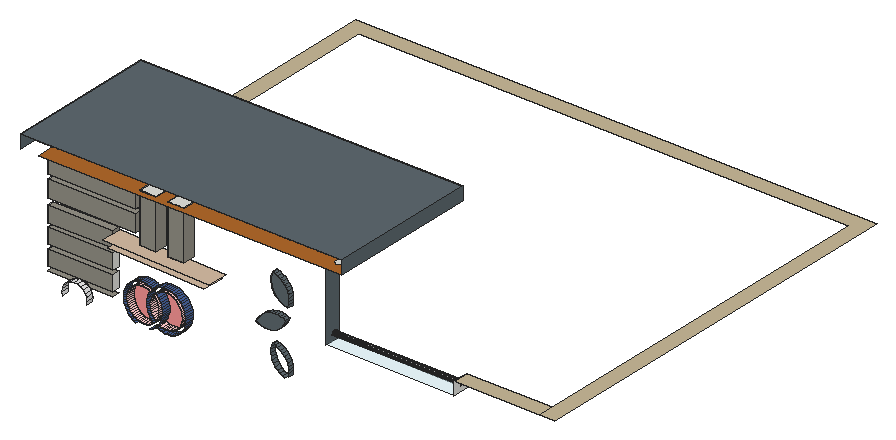
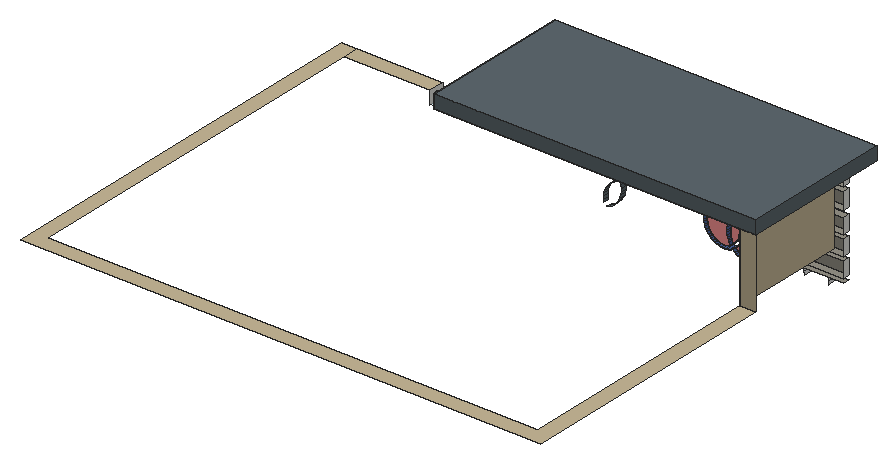
# SketchUp Ruby script. Lengths in inches.
U = 1.inch
M = Sketchup.active_model
def pt(a) = Geom::Point3d.new(a.map { |v| v * U })
def face(e, loops, mat)
  f = e.add_face(loops[0].map { |a| pt(a) })
  loops[1..].each { |l| e.add_face(l.map { |a| pt(a) }).erase! }
  f.material = f.back_material = mat if mat
  f
end
# faces: each face lists its corners as indices into pts; further lists are holes
def faces(e, pts, list, mat = nil) = list.each { |f| face(e, (f[0].is_a?(Array) ? f : [f]).map { |l| l.map { |i| pts[i] } }, mat) }
# xy, xz, yz: faces in a plane at the given z, y or x. An outline is a flat list of corners, or four numbers for a rectangle; further outlines are holes
def ring(l) = l.size == 4 ? [[l[0], l[1]], [l[2], l[1]], [l[2], l[3]], [l[0], l[3]]] : l.each_slice(2).to_a
def flat(e, list, mat, &to3) = list.each { |f| face(e, (f[0].is_a?(Array) ? f : [f]).map { |l| ring(l).map { |u, v| to3.(u, v) } }, mat) }
def xy(e, z, list, mat = nil) = flat(e, list, mat) { |x, y| [x, y, z] }
def xz(e, y, list, mat = nil) = flat(e, list, mat) { |x, z| [x, y, z] }
def yz(e, x, list, mat = nil) = flat(e, list, mat) { |y, z| [x, y, z] }
def lines(e, pts, list) = list.each { |a, b| e.add_line(pt(pts[a]), pt(pts[b])) }
# prism: a flat outline (further loops are holes) pulled along v
def prism(e, loops, v, mat = nil)
  f = face(e, loops, mat); d = Geom::Vector3d.new(v.map { |x| x * U })
  f.pushpull(f.normal.samedirection?(d) ? d.length : -d.length)
end
def box(e, o, s, mat = nil) = prism(e, [[o, [o[0] + s[0], o[1], o[2]], [o[0] + s[0], o[1] + s[1], o[2]], [o[0], o[1] + s[1], o[2]]]], [0, 0, s[2]], mat)
def at(x, y, z, deg = 0) = Geom::Transformation.translation(pt([x, y, z])) * Geom::Transformation.rotation(ORIGIN, Z_AXIS, deg.degrees)
def axes(o, x, y, z) = Geom::Transformation.new([*x, 0, *y, 0, *z, 0, *pt(o).to_a, 1])
def part(name) = M.definitions.add(name)
# library, detail: a bought-in or finely detailed component or shape, given as its bounding box
def library(name, o, s) = part(name).tap { |d| box(d.entities, o, s) }
def detail(e, o, s) = box(e.add_group.entities, o, s)
def put(e, d, t, mat = nil) = e.add_instance(d, t).tap { |i| i.material = mat if mat }
def group(e, t, mat = nil) = e.add_group.tap { |g| g.transformation = t; g.material = mat if mat }.entities
root = M.entities
M.materials.add("[Color A01]").color = [255, 204, 204]
M.materials.add("[Color A02]").color = [255, 153, 153]
M.materials.add("[Color M03]").color = [170, 170, 170]
M.materials.add("[Formica Blue]").color = [71, 97, 152]
M.materials.add("[Formica Graystone]").color = [149, 146, 135]
M.materials.add("[Formica Laminate Light]").color = [213, 189, 164]
M.materials.add("[Formica Speckled Grey]").color = [94, 105, 111]
M.materials.add("[Polished Concrete Old]").color = [229, 229, 229]
M.materials.add("[Quartz Light Brown]").color = [199, 184, 152]
M.materials.add("[Translucent Glass Safety]").color = [204, 235, 244]
M.materials["[Translucent Glass Safety]"].alpha = 0.5
M.materials.add("[Wood Bamboo]").color = [177, 105, 43]
xy(root,353.58,[[205.21,257.39,307.34,269.01]],"[Formica Graystone]")
xy(root,360.21,[[205.21,257.39,307.34,269.01]],"[Formica Graystone]")
xy(root,384.21,[[205.21,257.39,307.34,269.01]],"[Formica Graystone]")
xy(root,390.83,[[205.21,257.39,307.34,269.01]],"[Formica Graystone]")
xy(root,394.11,[[630.73,269.01,829.97,293.12]],"[Translucent Glass Safety]")
xy(root,414.1875,[[963.43,269.01,987.53,269.01,987.53,894.96,176.71,894.96,176.71,475.31,200.82,475.31,200.82,870.85,963.43,870.85],[829.97,269.01,963.43,293.12]],"[Quartz Light Brown]")
xy(root,414.83,[[205.21,257.39,307.34,269.01]],"[Formica Graystone]")
xy(root,415.78,[[556.52,261.14,561.09,269.01]],"[Formica Speckled Grey]")
xy(root,421.46,[[205.21,257.39,307.34,269.01]],"[Formica Graystone]")
xy(root,435.11,[[471.96,228.91,316.5,235.72,317.94,268.69,473.4,261.88]],"[Formica Laminate Light]")
xy(root,442.52,[[479.36,228.58,480.8,261.55,310.54,269.01,309.09,236.05]],"[Formica Laminate Light]")
xy(root,445.43,[[354.6875,249.89,380.1875,269.01],[399.125,249.89,424.625,269.01]])
xy(root,445.46,[[205.21,257.39,307.34,269.01]],"[Formica Graystone]")
xy(root,455.16,[[205.21,257.39,342.46,269.01]],"[Formica Graystone]")
xy(root,481.6,[[205.21,257.39,342.46,269.01]],"[Formica Graystone]")
xy(root,488.66,[[205.21,257.39,342.46,269.01]],"[Formica Graystone]")
xy(root,515.1,[[205.21,257.39,342.46,269.01]],"[Formica Graystone]")
xy(root,522.12,[[354.6875,249.89,380.1875,249.89,380.1875,269.01,399.125,269.01,399.125,249.89,424.625,249.89,424.625,269.01,630.73,269.01,630.73,293.12,200.82,293.12,200.82,475.31,176.71,475.31,176.71,269.01,354.6875,269.01],[657.37,255.45,655.28,255.73,653.34,256.53,651.67,257.8125,650.38,259.48,649.58,261.43,649.3,263.51,649.58,265.6,650.38,267.55,651.67,269.22,653.34,270.5,655.28,271.3,657.37,271.58,659.45,271.3,661.4,270.5,663.07,269.22,664.35,267.55,665.16,265.6,665.43,263.51,665.16,261.43,664.35,259.48,663.07,257.8125,661.4,256.53,659.45,255.73],[657.37,298.2,655.28,298.48,653.34,299.28,651.67,300.5625,650.38,302.23,649.58,304.18,649.3,306.26,649.58,308.35,650.38,310.3,651.67,311.97,653.34,313.25,655.28,314.05,657.37,314.33,659.45,314.05,661.4,313.25,663.07,311.97,664.35,310.3,665.16,308.35,665.43,306.26,665.16,304.18,664.35,302.23,663.07,300.5625,661.4,299.28,659.45,298.48],[657.37,359.33,655.28,359.6,653.34,360.41,651.67,361.6875,650.38,363.36,649.58,365.3,649.3,367.39,649.58,369.48,650.38,371.42,651.67,373.09,653.34,374.37,655.28,375.18,657.37,375.45,659.45,375.18,661.4,374.37,663.07,373.09,664.35,371.42,665.16,369.48,665.43,367.39,665.16,365.3,664.35,363.36,663.07,361.6875,661.4,360.41,659.45,359.6],[657.37,429.01,655.28,429.29,653.34,430.09,651.67,431.375,650.38,433.05,649.58,434.99,649.3,437.08,649.58,439.16,650.38,441.11,651.67,442.78,653.34,444.06,655.28,444.86,657.37,445.14,659.45,444.86,661.4,444.06,663.07,442.78,664.35,441.11,665.16,439.16,665.43,437.08,665.16,434.99,664.35,433.05,663.07,431.375,661.4,430.09,659.45,429.29]])
xy(root,522.12,[[[205.21,240.39,205.21,269.01,354.6875,269.01,354.6875,249.89,380.1875,249.89,380.1875,269.01,399.125,269.01,399.125,249.89,424.625,249.89,424.625,269.01,630.73,269.01,630.73,293.12,200.82,293.12,200.82,475.31,678.16,475.31,678.16,240.39],[657.37,255.45,659.45,255.73,661.4,256.53,663.07,257.8125,664.35,259.48,665.16,261.43,665.43,263.51,665.16,265.6,664.35,267.55,663.07,269.22,661.4,270.5,659.45,271.3,657.37,271.58,655.28,271.3,653.34,270.5,651.67,269.22,650.38,267.55,649.58,265.6,649.3,263.51,649.58,261.43,650.38,259.48,651.67,257.8125,653.34,256.53,655.28,255.73],[657.37,429.01,659.45,429.29,661.4,430.09,663.07,431.375,664.35,433.05,665.16,434.99,665.43,437.08,665.16,439.16,664.35,441.11,663.07,442.78,661.4,444.06,659.45,444.86,657.37,445.14,655.28,444.86,653.34,444.06,651.67,442.78,650.38,441.11,649.58,439.16,649.3,437.08,649.58,434.99,650.38,433.05,651.67,431.375,653.34,430.09,655.28,429.29],[657.37,298.2,659.45,298.48,661.4,299.28,663.07,300.5625,664.35,302.23,665.16,304.18,665.43,306.26,665.16,308.35,664.35,310.3,663.07,311.97,661.4,313.25,659.45,314.05,657.37,314.33,655.28,314.05,653.34,313.25,651.67,311.97,650.38,310.3,649.58,308.35,649.3,306.26,649.58,304.18,650.38,302.23,651.67,300.5625,653.34,299.28,655.28,298.48],[657.37,359.33,659.45,359.6,661.4,360.41,663.07,361.6875,664.35,363.36,665.16,365.3,665.43,367.39,665.16,369.48,664.35,371.42,663.07,373.09,661.4,374.37,659.45,375.18,657.37,375.45,655.28,375.18,653.34,374.37,651.67,373.09,650.38,371.42,649.58,369.48,649.3,367.39,649.58,365.3,650.38,363.36,651.67,361.6875,653.34,360.41,655.28,359.6]]],"[Wood Bamboo]")
xy(root,542.5625,[[176.71,240.39,678.16,475.31]],"[Formica Speckled Grey]")
xz(root,249.89,[[354.6875,445.43,380.1875,522.12],[399.125,445.43,424.625,522.12]],"[Formica Graystone]")
xz(root,257.39,[[241.74,353.58,242.42,354.47,246.48,357.59,251.2,359.54,256.27,360.21,261.34,359.54,266.07,357.59,270.125,354.47,270.81,353.58]])
xz(root,257.39,[[205.21,360.21,307.34,384.21],[205.21,390.83,307.34,414.83],[205.21,421.46,307.34,445.46],[205.21,455.16,342.46,481.6],[205.21,488.66,342.46,515.1]],"[Formica Graystone]")
xz(root,261.14,[[545.83,390.61,550.5625,391.09,555.16,392.3,559.51,394.21,563.5,396.78,567.05,399.94,570.07,403.61,572.47,407.71,574.21,412.13,570.02,413.94,565.61,415.16,561.09,415.78,556.52,415.78,551.99,415.17,547.59,413.96,543.39,412.17,539.47,409.82,535.9,406.98,532.74,403.67,530.06,399.98,527.89,395.95,532.01,393.57,536.44,391.87,541.09,390.87],[577.86,431.06,578.89,435.51,579.32,440.06,579.125,444.62,578.32,449.12,576.92,453.47,574.95,457.59,572.4375,461.4,569.4375,464.85,566,467.86,562.19,470.38,558.08,472.37,553.74,473.78,552.125,469.3125,551.23,464.64,551.07,459.89,551.65,455.18,552.96,450.61,554.97,446.3,557.62,442.36,560.86,438.88,564.59,435.95,568.74,433.63,573.2,431.99]],"[Formica Speckled Grey]")
xz(root,475.31,[[176.71,522.12,678.16,542.5625]],"[Formica Speckled Grey]")
xz(root,475.31,[[176.71,414.1875,200.82,522.12]],"[Quartz Light Brown]")
yz(root,176.71,[[240.39,522.12,475.31,542.5625]],"[Formica Speckled Grey]")
yz(root,200.82,[[293.12,414.1875,475.31,522.12]],"[Quartz Light Brown]")
yz(root,205.21,[[257.39,360.21,269.01,384.21],[257.39,390.83,269.01,414.83],[257.39,421.46,269.01,445.46],[257.39,455.16,269.01,481.6],[257.39,488.66,269.01,515.1]])
yz(root,307.34,[[257.39,360.21,269.01,384.21],[257.39,390.83,269.01,414.83]])
yz(root,307.34,[[257.39,421.46,269.01,445.46]],"[Formica Graystone]")
yz(root,342.46,[[257.39,455.16,269.01,481.6],[257.39,488.66,269.01,515.1]],"[Formica Graystone]")
yz(root,354.6875,[[249.89,445.43,269.01,522.12]],"[Formica Graystone]")
yz(root,380.1875,[[249.89,445.43,269.01,522.12]],"[Formica Graystone]")
yz(root,399.125,[[249.89,445.43,269.01,522.12]],"[Formica Graystone]")
yz(root,424.625,[[249.89,445.43,269.01,522.12]],"[Formica Graystone]")
yz(root,630.73,[[[269.01,394.11,293.12,522.12],[283.11,402.26,282.2,402.38,281.36,402.73,280.63,403.29,280.07,404.01,279.72,404.86,279.61,405.76,279.72,406.67,280.07,407.51,280.63,408.24,281.36,408.79,282.2,409.14,283.11,409.26,284.01,409.14,284.86,408.79,285.58,408.24,286.14,407.51,286.49,406.67,286.61,405.76,286.49,404.86,286.14,404.01,285.58,403.29,284.86,402.73,284.01,402.38]]],"[Formica Speckled Grey]")
yz(root,678.16,[[240.39,522.12,475.31,542.5625]],"[Formica Speckled Grey]")
yz(root,829.97,[[[269.01,394.11,293.12,414.1875],[283.11,402.26,284.01,402.38,284.86,402.73,285.58,403.29,286.14,404.01,286.49,404.86,286.61,405.76,286.49,406.67,286.14,407.51,285.58,408.24,284.86,408.79,284.01,409.14,283.11,409.26,282.2,409.14,281.36,408.79,280.63,408.24,280.07,407.51,279.72,406.67,279.61,405.76,279.72,404.86,280.07,404.01,280.63,403.29,281.36,402.73,282.2,402.38]]])
p = [[368.52,266.47,331.49],[371.5625,266.34,332.78],[371,253.35,332.78],[367.95,253.49,331.49],[568.74,269.01,333.44],[573.2,269.01,331.8],
  [573.2,261.14,331.8],[568.74,261.14,333.44],[342.88,267.6,333.33],[345.88,267.47,331.92],[345.31,254.48,331.92],[342.3125,254.61,333.33],
  [374.46,266.21,334.38],[373.89,253.23,334.38],[340.05,267.72,335.04],[339.48,254.73,335.04],[564.59,269.01,335.76],[564.59,261.14,335.76],
  [396.41,265.25,334.41],[399.7,265.11,334.69],[399.14,252.12,334.69],[395.84,252.26,334.41],[393.1,265.4,334.47],[392.53,252.41,334.47],
  [377.17,266.09,336.28],[376.6,253.11,336.28],[389.82,265.54,334.88],[389.25,252.55,334.88],[402.95,264.96,335.32],[402.38,251.98,335.32],
  [386.6,265.68,335.63],[386.03,252.69,335.63],[337.41,267.84,337.03],[336.84,254.85,337.03],[361.35,266.79,335.375],[358.63,266.91,335.14],
  [358.06,253.92,335.14],[360.78,253.8,335.375],[355.9,267.03,335.19],[355.33,254.04,335.19],[373.78,266.24,340.64],[375.08,266.1875,341.77],
  [375.01,266.1875,341.82],[372.6,266.3,344.08],[370.43,266.39,346.58],[368.54,266.47,349.3],[366.9375,266.54,352.2],[365.65,266.6,355.25],
  [364.6875,266.64,358.41],[364.0625,266.67,361.66],[363.78,266.68,364.96],[363.84,266.68,368.27],[364.25,266.66,371.56],[365,266.63,374.78],
  [366.08,266.58,377.91],[367.48,266.52,380.91],[369.19,266.44,383.74],[369.7,266.42,384.41],[367.5625,266.52,385.41],[364.99,266.63,386.31],
  [362.33,266.75,386.93],[359.62,266.86,387.26],[356.89,266.98,387.32],[354.17,267.1,387.08],[351.49,267.22,386.5625],[348.88,267.33,385.77],
  [346.36,267.44,384.71],[343.97,267.55,383.38],[341.74,267.65,381.82],[339.67,267.74,380.03],[337.81,267.82,378.04],[336.16,267.89,375.86],
  [334.75,267.95,373.52],[333.6,268,371.04],[332.7,268.04,368.46],[332.09,268.07,365.8],[331.75,268.09,363.09],[331.7,268.09,360.36],
  [331.93,268.08,357.64],[332.45,268.05,354.95],[333.24,268.02,352.34],[334.3,267.97,349.82],[335.62,267.92,347.43],[337.18,267.85,345.19],
  [338.97,267.77,343.125],[340.97,267.68,341.26],[343.14,267.59,339.61],[345.48,267.48,338.2],[347.95,267.375,337.04],[350.53,267.26,336.15],
  [353.19,267.15,335.53],[364.03,266.67,335.89],[366.64,266.56,336.6875],[369.15,266.45,337.75],[371.54,266.34,339.07],[352.62,254.16,335.53],
  [406.12,264.83,336.28],[405.55,251.84,336.28],[578.89,269.01,335.32],[579.32,269.01,339.87],[579.32,261.14,339.87],[578.89,261.14,335.32],
  [363.46,253.68,335.89],[349.96,254.27,336.15],[236.6875,257.39,340.62],[237.35,257.39,335.55],[237.35,246.45,335.55],[236.6875,246.45,340.62],
  [275.19,257.39,335.55],[275.86,257.39,340.62],[275.86,246.45,340.62],[275.19,246.45,335.55],[383.48,265.82,336.71],[382.91,252.83,336.71],
  [560.86,269.01,338.69],[560.86,261.14,338.69],[366.07,253.57,336.6875],[347.38,254.39,337.04],[409.16,264.69,337.57],[408.59,251.71,337.57],
  [379.67,265.99,338.44],[379.1,253,338.44],[380.48,265.95,338.12],[379.91,252.96,338.12],[368.58,253.46,337.75],[344.91,254.5,338.2],
  [335,267.94,339.3],[334.43,254.96,339.3],[412.06,264.57,339.17],[411.49,251.58,339.17],[370.97,253.35,339.07],[379.77,265.98,338.55],
  [379.2,252.99,338.55],[342.57,254.6,339.61],[557.62,269.01,342.17],[557.62,261.14,342.17],[373.21,253.26,340.64],[414.77,264.45,341.0625],
  [414.2,251.46,341.0625],[332.83,268.04,341.8],[332.26,255.05,341.8],[340.4,254.69,341.26],[398.95,265.14,340.16],[396.23,265.26,339.93],
  [395.66,252.27,339.93],[398.375,252.15,340.16],[393.5,265.38,339.98],[392.93,252.39,339.98],[579.125,269.01,344.43],[579.125,261.14,344.43],
  [383.92,265.8,343.5],[383.42,265.82,342.83],[385.55,265.73,341.83],[388.13,265.61,340.9375],[390.79,265.5,340.32],[401.625,265.02,340.68],
  [404.24,264.91,341.47],[406.75,264.8,342.54],[409.14,264.69,343.86],[411.38,264.6,345.42],[413.44,264.51,347.21],[415.31,264.42,349.21],
  [416.95,264.35,351.39],[418.36,264.29,353.73],[419.52,264.24,356.2],[420.41,264.2,358.78],[421.03,264.17,361.44],[421.37,264.16,364.15],
  [421.42,264.16,366.89],[421.18,264.17,369.61],[420.67,264.1875,372.29],[419.875,264.22,374.9],[418.8125,264.27,377.42],[417.49,264.33,379.8125],
  [415.93,264.4,382.05],[414.14,264.47,384.12],[412.15,264.5625,385.98],[409.97,264.66,387.63],[407.63,264.76,389.04],[405.16,264.87,390.2],
  [402.58,264.98,391.09],[399.92,265.1,391.71],[397.22,265.22,392.05],[394.49,265.34,392.1],[391.77,265.46,391.87],[389.09,265.57,391.35],
  [386.48,265.6875,390.56],[383.96,265.8,389.49],[381.57,265.9,388.17],[379.33,266,386.61],[378.03,266.06,385.48],[378.1,266.05,385.42],
  [380.52,265.95,383.16],[382.6875,265.85,380.66],[384.58,265.77,377.95],[386.18,265.7,375.05],[387.46,265.64,372],[388.43,265.6,368.83],
  [389.05,265.57,365.58],[389.34,265.5625,362.28],[389.27,265.5625,358.97],[388.86,265.58,355.6875],[388.12,265.62,352.46],[387.03,265.66,349.34],
  [385.63,265.72,346.34],[390.22,252.51,340.32],[401.06,252.04,340.68],[387.5625,252.625,340.9375],[237.35,257.39,345.69],[237.35,246.45,345.69],
  [275.19,257.39,345.69],[275.19,246.45,345.69],[374.51,253.2,341.77],[403.67,251.92,341.47],[384.98,252.74,341.83],[417.27,264.34,343.23],
  [416.7,251.35,343.23],[338.4,254.78,343.125],[406.18,251.8125,342.54],[382.85,252.83,342.83],[374.44,253.2,341.82],[372.03,253.31,344.08],
  [330.9375,268.12,344.51],[330.37,255.13,344.51],[554.97,269.01,346.12],[554.97,261.14,346.12],[408.57,251.71,343.86],[383.35,252.8125,343.5],
  [336.62,254.86,345.19],[419.53,264.24,345.65],[418.96,251.25,345.65],[385.0625,252.74,346.34],[410.81,251.61,345.42],[369.86,253.4,346.58],
  [578.32,269.01,348.93],[578.32,261.14,348.93],[329.34,268.19,347.41],[328.77,255.2,347.41],[335.05,254.93,347.43],[412.87,251.52,347.21],
  [421.52,264.15,348.29],[420.95,251.16,348.29],[239.3125,257.39,350.42],[239.3125,246.45,350.42],[273.24,257.39,350.42],[273.24,246.45,350.42],
  [378.8,266.02,345.87],[378.5625,266.03,346.05],[377.99,253.05,346.05],[378.23,253.04,345.87],[379.35,266,346.6],[378.78,253.01,346.6],
  [374.55,266.21,381.2],[374.3125,266.22,381.375],[373.76,266.24,380.64],[372.35,266.31,378.3],[371.19,266.36,375.83],[370.3,266.4,373.25],
  [369.68,266.42,370.59],[369.35,266.4375,367.875],[369.29,266.44,365.15],[369.53,266.43,362.42],[370.05,266.41,359.74],[370.84,266.37,357.125],
  [371.9,266.33,354.61],[373.22,266.27,352.22],[374.78,266.2,349.98],[376.57,266.12,347.91],[380.76,265.9375,348.9375],[381.92,265.89,351.41],
  [382.8125,265.85,353.99],[383.43,265.82,356.66],[383.77,265.81,359.37],[383.82,265.8,362.1],[383.59,265.8125,364.82],[383.07,265.84,367.5],
  [382.28,265.87,370.12],[381.21,265.92,372.63],[379.89,265.98,375.03],[378.33,266.04,377.27],[376.54,266.12,379.33],[376,253.13,347.91],
  [552.96,269.01,350.42],[552.96,261.14,350.42],[386.46,252.67,349.34],[380.19,252.95,348.9375],[367.97,253.49,349.3],[414.74,251.4375,349.21],
  [333.73,254.99,349.82],[328.05,268.25,350.46],[327.48,255.26,350.46],[374.21,253.21,349.98],[423.23,264.08,351.125],[422.66,251.09,351.125],
  [381.35,252.9,351.41],[576.92,269.01,353.28],[576.92,261.14,353.28],[416.38,251.36,351.39],[387.55,252.63,352.46],[366.37,253.56,352.2],
  [332.67,255.03,352.34],[372.65,253.28,352.22],[242.42,257.39,354.47],[241.74,257.39,353.58],[241.74,246.45,353.58],[242.42,246.45,354.47],
  [270.81,257.39,353.58],[270.125,257.39,354.47],[270.125,246.45,354.47],[270.81,246.45,353.58],[551.65,269.01,354.99],[551.65,261.14,354.99],
  [327.09,268.29,353.625],[326.52,255.3,353.625],[424.63,264.01,354.12],[424.0625,251.03,354.12],[417.79,251.3,353.73],[382.24,252.86,353.99],
  [371.33,253.34,354.61],[365.08,253.61,355.25],[331.88,255.07,354.95],[388.3,252.59,355.6875],[574.95,269.01,357.4],[574.95,261.14,357.4],
  [326.46,268.32,356.875],[325.9,255.33,356.875],[418.95,251.25,356.2],[382.86,252.83,356.66],[425.71,263.97,357.25],[425.14,250.98,357.25],
  [246.48,257.39,357.59],[246.48,246.45,357.59],[266.07,257.39,357.59],[266.07,246.45,357.59],[370.27,253.38,357.125],[331.36,255.09,357.64],
  [551.07,269.01,359.71],[551.07,261.14,359.71],[364.12,253.65,358.41],[388.7,252.58,358.97],[419.84,251.21,358.78],[383.2,252.82,359.37],
  [326.18,268.33,360.17],[325.61,255.34,360.17],[369.48,253.42,359.74],[426.46,263.93,360.48],[425.89,250.95,360.48],[572.4375,269.01,361.21],
  [572.4375,261.14,361.21],[251.2,257.39,359.54],[251.2,246.45,359.54],[261.34,257.39,359.54],[261.34,246.45,359.54],[331.13,255.1,360.36],
  [363.49,253.68,361.66],[420.46,251.19,361.44],[388.77,252.57,362.28],[383.25,252.82,362.1],[256.27,257.39,360.21],[256.27,246.45,360.21],
  [368.96,253.44,362.42],[551.23,269.01,364.46],[551.23,261.14,364.46],[326.24,268.33,363.48],[325.67,255.34,363.48],[331.18,255.1,363.09],
  [426.87,263.92,363.76],[426.3,250.93,363.76],[569.4375,269.01,364.66],[569.4375,261.14,364.66],[420.8,251.17,364.15],[363.21,253.69,364.96],
  [383.02,252.83,364.82],[388.48,252.59,365.58],[368.73,253.45,365.15],[331.52,255.08,365.8],[326.65,268.31,366.77],[326.08,255.32,366.77],
  [426.93,263.91,367.07],[426.36,250.93,367.07],[420.85,251.17,366.89],[552.125,269.01,369.125],[552.125,261.14,369.125],[566,269.01,367.67],
  [566,261.14,367.67],[382.5,252.85,367.5],[363.27,253.69,368.27],[368.78,253.45,367.875],[387.86,252.61,368.83],[332.13,255.06,368.46],
  [327.4,268.28,369.99],[326.83,255.29,369.99],[420.62,251.18,369.61],[426.65,263.93,370.37],[426.08,250.9375,370.37],[381.71,252.88,370.12],
  [562.19,269.01,370.19],[562.19,261.14,370.19],[369.11,253.44,370.59],[363.68,253.67,371.56],[333.03,255.02,371.04],[386.9,252.66,372],
  [553.74,269.01,373.59],[553.74,261.14,373.59],[420.1,251.2,372.29],[328.48,268.23,373.12],[327.91,255.24,373.12],[380.64,252.93,372.63],
  [558.08,269.01,372.18],[558.08,261.14,372.18],[426.02,263.95,373.62],[425.46,250.97,373.62],[369.73,253.41,373.25],[334.18,254.97,373.52],
  [364.43,253.64,374.78],[385.61,252.71,375.05],[419.3,251.24,374.9],[379.32,252.99,375.03],[329.89,268.17,376.12],[329.32,255.18,376.12],
  [370.625,253.37,375.83],[335.59,254.9,375.86],[425.0625,264,376.79],[424.49,251.01,376.79],[365.51,253.59,377.91],[418.24,251.28,377.42],
  [384.01,252.78,377.95],[377.76,253.06,377.27],[371.78,253.32,378.3],[337.24,254.83,378.04],[331.59,268.09,378.95],[331.02,255.1,378.95],
  [423.78,264.05,379.83],[423.21,251.06,379.83],[375.98,253.13,379.33],[416.92,251.34,379.8125],[382.12,252.87,380.66],[366.91,253.53,380.91],
  [339.1,254.75,380.03],[373.19,253.26,380.64],[333.59,268,381.59],[333.02,255.02,381.59],[373.98,253.22,381.2],[422.18,264.12,382.73],
  [421.61,251.13,382.73],[415.36,251.41,382.05],[341.17,254.66,381.82],[373.74,253.23,381.375],[379.95,252.96,383.16],[368.62,253.46,383.74],
  [335.85,267.91,384.01],[335.28,254.92,384.01],[343.41,254.5625,383.38],[413.57,251.49,384.12],[420.28,264.21,385.45],[419.71,251.22,385.45],
  [377.54,253.07,385.42],[345.79,254.46,384.71],[369.13,253.43,384.41],[338.35,267.8,386.18],[337.78,254.81,386.18],[411.58,251.57,385.98],
  [367,253.53,385.41],[348.31,254.35,385.77],[418.12,264.3,387.95],[417.55,251.3125,387.95],[377.46,253.07,385.48],[364.42,253.64,386.31],
  [378.77,253.01,386.61],[350.92,254.23,386.5625],[409.4,251.67,387.63],[341.06,267.68,388.07],[340.49,254.69,388.07],[361.76,253.76,386.93],
  [381,252.91,388.17],[353.6,254.12,387.08],[359.05,253.875,387.26],[356.32,254,387.32],[407.07,251.77,389.04],[415.7,264.41,390.21],
  [415.13,251.42,390.21],[343.95,267.55,389.67],[343.38,254.5625,389.67],[383.39,252.81,389.49],[373.35,266.26,388.7],[372.63,266.29,389.13],
  [372.07,253.31,389.13],[372.78,253.27,388.7],[373.44,266.26,388.8],[372.875,253.27,388.8],[375.94,266.15,390.97],[375.375,253.16,390.97],
  [404.59,251.88,390.2],[369.64,266.42,390.53],[369.07,253.4375,390.53],[385.91,252.7,390.56],[347,267.42,390.96],[346.43,254.43,390.96],
  [413.06,264.52,392.21],[412.5,251.53,392.21],[402.01,251.99,391.09],[366.51,266.5625,391.61],[365.95,253.57,391.61],[388.52,252.58,391.35],
  [541.09,269.01,390.87],[545.83,269.01,390.61],[545.83,261.14,390.61],[541.09,261.14,390.87],[550.5625,269.01,391.09],[550.5625,261.14,391.09],
  [536.44,269.01,391.87],[536.44,261.14,391.87],[378.66,266.03,392.86],[378.09,253.04,392.86],[350.16,267.28,391.93],[349.59,254.29,391.93],
  [399.36,252.11,391.71],[555.16,269.01,392.3],[555.16,261.14,392.3],[391.2,252.47,391.87],[363.29,266.7,392.36],[362.72,253.72,392.36],
  [396.65,252.23,392.05],[393.92,252.35,392.1],[353.41,267.14,392.55],[352.84,254.15,392.55],[532.01,269.01,393.57],[532.01,261.14,393.57],
  [410.23,264.65,393.92],[409.66,251.66,393.92],[559.51,269.01,394.21],[559.51,261.14,394.21],[360.01,266.85,392.77],[359.44,253.86,392.77],
  [356.7,266.99,392.84],[356.14,254,392.84],[381.55,265.9,394.46],[380.98,252.92,394.46],[527.89,269.01,395.95],[527.89,261.14,395.95],
  [407.24,264.78,395.32],[406.67,251.79,395.32],[563.5,269.01,396.78],[563.5,261.14,396.78],[384.6,265.77,395.75],[384.03,252.78,395.75],
  [404.11,264.91,396.4],[403.54,251.93,396.4],[387.76,265.63,396.71],[387.19,252.64,396.71],[530.06,269.01,399.98],[530.06,261.14,399.98],
  [400.89,265.06,397.15],[400.32,252.07,397.15],[391.01,265.49,397.34],[390.4375,252.5,397.34],[567.05,269.01,399.94],[567.05,261.14,399.94],
  [397.61,265.2,397.56],[397.04,252.21,397.56],[394.3,265.34,397.62],[393.73,252.36,397.62],[570.07,269.01,403.61],[570.07,261.14,403.61],
  [532.74,269.01,403.67],[532.74,261.14,403.67],[829.97,283.11,402.26],[829.97,282.2,402.38],[630.73,282.2,402.38],[630.73,283.11,402.26],
  [829.97,284.01,402.38],[630.73,284.01,402.38],[829.97,281.36,402.73],[630.73,281.36,402.73],[829.97,284.86,402.73],[630.73,284.86,402.73],
  [829.97,280.63,403.29],[630.73,280.63,403.29],[829.97,285.58,403.29],[630.73,285.58,403.29],[829.97,280.07,404.01],[630.73,280.07,404.01],
  [829.97,286.14,404.01],[630.73,286.14,404.01],[572.47,269.01,407.71],[572.47,261.14,407.71],[535.9,269.01,406.98],[535.9,261.14,406.98],
  [829.97,279.72,404.86],[630.73,279.72,404.86],[829.97,286.49,404.86],[630.73,286.49,404.86],[829.97,279.61,405.76],[630.73,279.61,405.76],
  [829.97,286.61,405.76],[630.73,286.61,405.76],[829.97,279.72,406.67],[630.73,279.72,406.67],[829.97,286.49,406.67],[630.73,286.49,406.67],
  [829.97,280.07,407.51],[630.73,280.07,407.51],[829.97,286.14,407.51],[630.73,286.14,407.51],[539.47,269.01,409.82],[539.47,261.14,409.82],
  [829.97,280.63,408.24],[630.73,280.63,408.24],[829.97,285.58,408.24],[630.73,285.58,408.24],[574.21,269.01,412.13],[574.21,261.14,412.13],
  [829.97,281.36,408.79],[630.73,281.36,408.79],[829.97,284.86,408.79],[630.73,284.86,408.79],[829.97,282.2,409.14],[630.73,282.2,409.14],
  [829.97,284.01,409.14],[630.73,284.01,409.14],[829.97,283.11,409.26],[630.73,283.11,409.26],[543.39,269.01,412.17],[543.39,261.14,412.17],
  [570.02,269.01,413.94],[570.02,261.14,413.94],[547.59,269.01,413.96],[547.59,261.14,413.96],[565.61,269.01,415.16],[565.61,261.14,415.16],
  [551.99,269.01,415.17],[551.99,261.14,415.17],[556.52,269.01,415.78],[556.52,261.14,415.78],[561.09,269.01,415.78],[561.09,261.14,415.78],
  [573.2,269.01,431.99],[577.86,269.01,431.06],[577.86,261.14,431.06],[573.2,261.14,431.99],[578.89,269.01,435.51],[578.89,261.14,435.51],
  [568.74,269.01,433.63],[568.74,261.14,433.63],[564.59,269.01,435.95],[564.59,261.14,435.95],[579.32,269.01,440.06],[579.32,261.14,440.06],
  [560.86,269.01,438.88],[560.86,261.14,438.88],[557.62,269.01,442.36],[557.62,261.14,442.36],[579.125,269.01,444.62],[579.125,261.14,444.62],
  [554.97,269.01,446.3],[554.97,261.14,446.3],[578.32,269.01,449.12],[578.32,261.14,449.12],[552.96,269.01,450.61],[552.96,261.14,450.61],
  [576.92,269.01,453.47],[576.92,261.14,453.47],[551.65,269.01,455.18],[551.65,261.14,455.18],[574.95,269.01,457.59],[574.95,261.14,457.59],
  [551.07,269.01,459.89],[551.07,261.14,459.89],[572.4375,269.01,461.4],[572.4375,261.14,461.4],[551.23,269.01,464.64],[551.23,261.14,464.64],
  [569.4375,269.01,464.85],[569.4375,261.14,464.85],[552.125,269.01,469.3125],[552.125,261.14,469.3125],[566,269.01,467.86],[566,261.14,467.86],
  [562.19,269.01,470.38],[562.19,261.14,470.38],[553.74,269.01,473.78],[553.74,261.14,473.78],[558.08,269.01,472.37],[558.08,261.14,472.37]]
faces(root,p,[[0,1,2,3],[8,9,10,11],[1,12,13,2],[14,8,11,15],[18,19,20,21],[22,18,21,23],[12,24,25,13],[26,22,23,27],
  [19,28,29,20],[30,26,27,31],[32,14,15,33],[28,96,97,29],[112,30,31,113],[96,118,119,97],[24,120,121,25],[122,112,113,123],
  [126,32,33,127],[118,128,129,119],[131,122,123,132],[120,131,132,121],[128,137,138,129],[139,126,127,140],[137,215,216,138],[43,42,220,221],
  [42,41,212,220],[222,139,140,223],[151,150,227,219],[215,229,230,216],[150,204,231,227],[44,43,221,233],[236,222,223,237],[229,240,241,230],
  [204,203,284,231],[45,44,233,286],[289,236,237,290],[240,292,293,241],[203,202,298,284],[46,45,286,299],[312,289,290,313],[292,314,315,293],
  [47,46,299,319],[202,201,321,298],[324,312,313,325],[314,328,329,315],[48,47,319,338],[201,200,339,321],[342,324,325,343],[328,345,346,329],
  [49,48,338,354],[200,199,356,339],[363,342,343,364],[345,366,367,346],[50,49,354,371],[199,198,373,356],[376,363,364,377],[366,378,379,367],
  [51,50,371,386],[198,197,388,373],[390,376,377,391],[378,393,394,379],[52,51,386,399],[197,196,401,388],[405,390,391,406],[393,410,411,394],
  [53,52,399,414],[196,195,415,401],[418,405,406,419],[410,422,423,411],[54,53,414,424],[195,194,426,415],[430,418,419,431],[422,432,433,423],
  [194,193,436,426],[55,54,424,437],[440,430,431,441],[432,443,444,433],[193,192,448,436],[56,55,437,449],[450,440,441,451],[443,454,455,444],
  [192,191,456,448],[57,56,449,458],[459,450,451,460],[454,464,465,455],[191,190,466,456],[471,459,460,472],[464,479,480,465],[481,471,472,482],
  [484,485,486,487],[488,484,487,489],[490,488,489,491],[485,493,494,486],[496,481,482,497],[479,498,499,480],[493,501,502,494],[512,490,491,513],
  [514,496,497,515],[501,520,521,502],[524,514,515,525],[498,528,529,499],[520,532,533,521],[534,524,525,535],[532,534,535,533],[536,512,513,537],
  [528,540,541,529],[544,536,537,545],[540,546,547,541],[548,544,545,549],[546,552,553,547],[554,548,549,555],[552,558,559,553],[560,554,555,561],
  [558,560,561,559]],"[Formica Blue]")
faces(root,p,[[4,5,6,7],[16,4,7,17],[98,99,100,101],[114,16,17,115],[134,114,115,135],[99,148,149,100],[224,134,135,225],[148,234,235,149],
  [282,224,225,283],[234,295,296,235],[310,282,283,311],[295,322,323,296],[336,310,311,337],[322,347,348,323],[361,336,337,362],[347,368,369,348],
  [381,361,362,382],[368,383,384,369],[383,396,397,384],[402,381,382,403],[396,408,409,397],[408,402,403,409],[504,505,506,507],[505,508,509,506],
  [510,504,507,511],[508,517,518,509],[526,510,511,527],[517,530,531,518],[538,526,527,539],[530,542,543,531],[550,538,539,551],[542,556,557,543],
  [556,562,563,557],[564,550,551,565],[562,584,585,563],[586,564,565,587],[604,586,587,605],[584,610,611,585],[622,604,605,623],[610,624,625,611],
  [626,622,623,627],[624,628,629,625],[630,626,627,631],[632,630,631,633],[628,634,635,629],[636,637,638,639],[637,640,641,638],[642,636,639,643],
  [644,642,643,645],[640,646,647,641],[648,644,645,649],[650,648,649,651],[646,652,653,647],[654,650,651,655],[652,656,657,653],[658,654,655,659],
  [656,660,661,657],[662,658,659,663],[660,664,665,661],[666,662,663,667],[664,668,669,665],[670,666,667,671],[668,672,673,669],[674,670,671,675],
  [672,676,677,673],[676,678,679,677],[680,674,675,681],[678,682,683,679],[682,680,681,683]],"[Formica Speckled Grey]")
faces(root,p,[[34,35,36,37],[35,38,39,36],[38,90,95,39],[91,34,37,102],[90,89,103,95],[92,91,102,116],[89,88,117,103],[93,92,116,124],
  [88,87,125,117],[94,93,124,130],[87,86,133,125],[40,94,130,136],[86,85,141,133],[142,143,144,145],[143,146,147,144],[146,154,205,147],
  [155,142,145,206],[154,153,207,205],[41,40,136,212],[156,155,206,213],[153,152,214,207],[85,84,217,141],[157,156,213,218],[152,151,219,214],
  [158,157,218,226],[84,83,228,217],[159,158,226,232],[83,82,238,228],[160,159,232,239],[246,247,248,249],[250,246,249,251],[247,267,281,248],
  [268,250,251,285],[161,160,239,287],[82,81,288,238],[267,266,291,281],[269,268,285,294],[162,161,287,297],[81,80,300,288],[266,265,301,291],
  [163,162,297,316],[270,269,294,317],[265,264,318,301],[80,79,320,300],[164,163,316,326],[271,270,317,327],[264,263,334,318],[79,78,335,320],
  [165,164,326,340],[272,271,327,341],[263,262,344,334],[78,77,353,335],[166,165,340,355],[273,272,341,357],[262,261,360,344],[77,76,365,353],
  [167,166,355,370],[274,273,357,372],[261,260,374,360],[76,75,375,365],[168,167,370,380],[275,274,372,385],[260,259,387,374],[75,74,389,375],
  [169,168,380,392],[276,275,385,395],[259,258,398,387],[74,73,400,389],[170,169,392,404],[277,276,395,407],[258,257,412,398],[73,72,413,400],
  [171,170,404,416],[278,277,407,417],[257,256,420,412],[72,71,421,413],[172,171,416,425],[279,278,417,427],[256,255,428,420],[71,70,429,421],
  [280,279,427,434],[173,172,425,435],[70,69,438,429],[255,254,439,428],[252,280,434,442],[174,173,435,445],[69,68,446,438],[254,253,447,439],
  [253,252,442,447],[68,67,452,446],[175,174,445,453],[67,66,457,452],[176,175,453,461],[58,57,458,462],[66,65,463,457],[59,58,462,467],
  [190,189,468,466],[65,64,469,463],[177,176,461,470],[60,59,467,473],[189,188,474,468],[64,63,475,469],[61,60,473,476],[63,62,477,475],
  [62,61,476,477],[178,177,470,478],[188,187,483,474],[179,178,478,492],[187,186,495,483],[180,179,492,500],[186,185,503,495],[181,180,500,516],
  [185,184,519,503],[182,181,516,522],[184,183,523,519],[183,182,522,523]],"[Color A01]")
faces(root,p,[[40,41,42,43,44,45,46,47,48,49,50,51,52,53,54,55,56,57,58,59,60,61,62,63,64,65,66,67,68,69,70,71,72,73,74,75,76,77,78,79,80,81,82,83,84,85,86,87,88,89,90,38,35,34,91,92,93,94],[150,151,152,153,154,146,143,142,155,156,157,158,159,160,161,162,163,164,165,166,167,168,169,170,171,172,173,174,175,176,177,178,179,180,181,182,183,184,185,186,187,188,189,190,191,192,193,194,195,196,197,198,199,200,201,202,203,204],[252,253,254,255,256,257,258,259,260,261,262,263,264,265,266,267,247,246,250,268,269,270,271,272,273,274,275,276,277,278,279,280]],"[Color A02]")
faces(root,p,[[104,105,106,107],[108,109,110,111],[208,104,107,209],[109,210,211,110],[242,208,209,243],[210,244,245,211],[302,303,242,243,304,305],[244,306,307,308,309,245],
  [330,302,305,331],[307,332,333,308],[349,330,331,350],[332,351,352,333],[358,349,350,359],[351,358,359,352]],"[Polished Concrete Old]")
faces(root,p,[[566,567,568,569],[570,566,569,571],[567,572,573,568],[574,570,571,575],[572,576,577,573],[578,574,575,579],[576,580,581,577],[582,578,579,583],
  [580,588,589,581],[590,582,583,591],[588,592,593,589],[594,590,591,595],[592,596,597,593],[598,594,595,599],[596,600,601,597],[602,598,599,603],
  [600,606,607,601],[608,602,603,609],[606,612,613,607],[614,608,609,615],[612,616,617,613],[618,614,615,619],[616,620,621,617],[620,618,619,621]],"[Color M03]")
